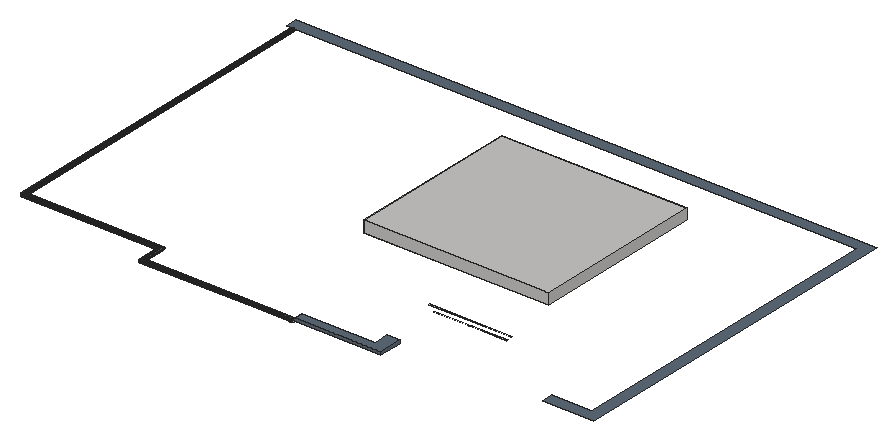
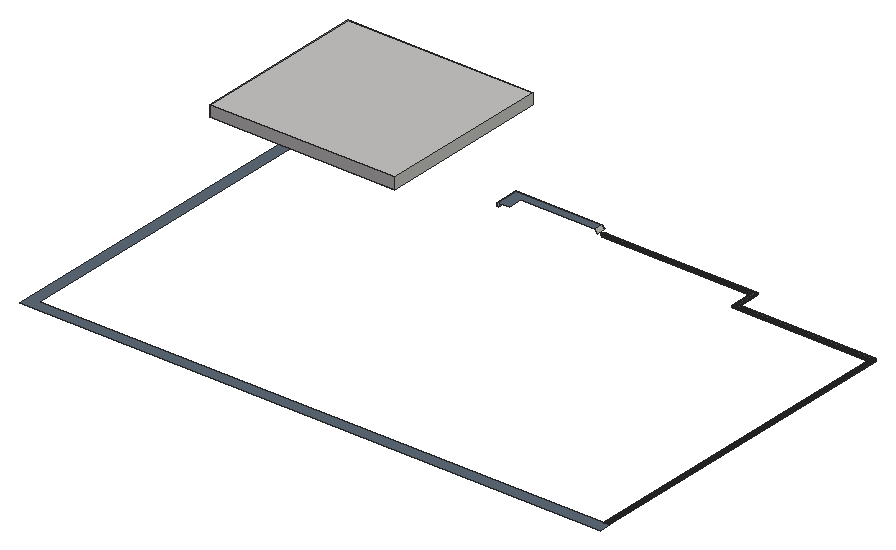
# SketchUp Ruby script. Lengths in inches.
U = 1.inch
M = Sketchup.active_model
def pt(a) = Geom::Point3d.new(a.map { |v| v * U })
def face(e, loops, mat)
  f = e.add_face(loops[0].map { |a| pt(a) })
  loops[1..].each { |l| e.add_face(l.map { |a| pt(a) }).erase! }
  f.material = f.back_material = mat if mat
  f
end
# faces: each face lists its corners as indices into pts; further lists are holes
def faces(e, pts, list, mat = nil) = list.each { |f| face(e, (f[0].is_a?(Array) ? f : [f]).map { |l| l.map { |i| pts[i] } }, mat) }
# xy, xz, yz: faces in a plane at the given z, y or x. An outline is a flat list of corners, or four numbers for a rectangle; further outlines are holes
def ring(l) = l.size == 4 ? [[l[0], l[1]], [l[2], l[1]], [l[2], l[3]], [l[0], l[3]]] : l.each_slice(2).to_a
def flat(e, list, mat, &to3) = list.each { |f| face(e, (f[0].is_a?(Array) ? f : [f]).map { |l| ring(l).map { |u, v| to3.(u, v) } }, mat) }
def xy(e, z, list, mat = nil) = flat(e, list, mat) { |x, y| [x, y, z] }
def xz(e, y, list, mat = nil) = flat(e, list, mat) { |x, z| [x, y, z] }
def yz(e, x, list, mat = nil) = flat(e, list, mat) { |y, z| [x, y, z] }
def lines(e, pts, list) = list.each { |a, b| e.add_line(pt(pts[a]), pt(pts[b])) }
# prism: a flat outline (further loops are holes) pulled along v
def prism(e, loops, v, mat = nil)
  f = face(e, loops, mat); d = Geom::Vector3d.new(v.map { |x| x * U })
  f.pushpull(f.normal.samedirection?(d) ? d.length : -d.length)
end
def box(e, o, s, mat = nil) = prism(e, [[o, [o[0] + s[0], o[1], o[2]], [o[0] + s[0], o[1] + s[1], o[2]], [o[0], o[1] + s[1], o[2]]]], [0, 0, s[2]], mat)
def at(x, y, z, deg = 0) = Geom::Transformation.translation(pt([x, y, z])) * Geom::Transformation.rotation(ORIGIN, Z_AXIS, deg.degrees)
def axes(o, x, y, z) = Geom::Transformation.new([*x, 0, *y, 0, *z, 0, *pt(o).to_a, 1])
def part(name) = M.definitions.add(name)
# library, detail: a bought-in or finely detailed component or shape, given as its bounding box
def library(name, o, s) = part(name).tap { |d| box(d.entities, o, s) }
def detail(e, o, s) = box(e.add_group.entities, o, s)
def put(e, d, t, mat = nil) = e.add_instance(d, t).tap { |i| i.material = mat if mat }
def group(e, t, mat = nil) = e.add_group.tap { |g| g.transformation = t; g.material = mat if mat }.entities
root = M.entities
M.materials.add("[0010_Snow]").color = [198, 195, 195]
M.materials.add("[0040_Peru]").color = [191, 124, 58]
M.materials.add("[0111_SlateGray]").color = [93, 106, 119]
xy(root,726,[[864,63,948,63,948,639,0,639,0,621,930,621,930,81,864,81]],"[0111_SlateGray]")
xy(root,726.875,[[485.39,25,485.39,27,627.8125,27,627.8125,63,629.8125,63,629.8125,25]],"[0111_SlateGray]")
xy(root,732,[[489.79,25,629.8125,25,629.8125,63,609.8125,63,609.8125,39,489.79,39]],"[0111_SlateGray]")
xy(root,793.97,[[687,62,746.59,63],[746.59,62,806.18,63]])
xy(root,801.97,[[679,62,814.18,63]])
xy(root,882,[[668.51,51.99,667.48,52.125,666.51,52.53,665.68,53.16,665.05,53.99,664.65,54.96,664.51,55.99,664.65,57.03,665.05,57.99,665.68,58.82,666.51,59.45,667.48,59.85,668.51,59.99,669.55,59.85,670.51,59.45,671.34,58.82,671.97,57.99,672.375,57.03,672.51,55.99,672.375,54.96,671.97,53.99,671.34,53.16,670.51,52.53,669.55,52.125],[728.51,51.99,727.48,52.125,726.51,52.53,725.68,53.16,725.05,53.99,724.65,54.96,724.51,55.99,724.65,57.03,725.05,57.99,725.68,58.82,726.51,59.45,727.48,59.85,728.51,59.99,729.55,59.85,730.51,59.45,731.34,58.82,731.97,57.99,732.375,57.03,732.51,55.99,732.375,54.96,731.97,53.99,731.34,53.16,730.51,52.53,729.55,52.125],[788.51,51.99,787.48,52.125,786.51,52.53,785.68,53.16,785.05,53.99,784.65,54.96,784.51,55.99,784.65,57.03,785.05,57.99,785.68,58.82,786.51,59.45,787.48,59.85,788.51,59.99,789.55,59.85,790.51,59.45,791.34,58.82,791.97,57.99,792.375,57.03,792.51,55.99,792.375,54.96,791.97,53.99,791.34,53.16,790.51,52.53,789.55,52.125],[609.8125,63,609.8125,303,621.8125,303,621.8125,81,852,81,852,303,864,303,864,63],[874.9375,71.95,873.375,72.05,871.89,72.55,870.59,73.42,869.55,74.59,868.86,76,868.55,77.53,868.65,79.09,869.15,80.58,870.01,81.88,871.1875,82.92,872.59,83.61,874.13,83.92,875.69,83.82,877.18,83.32,878.48,82.46,879.51,81.28,880.21,79.875,880.52,78.34,880.42,76.78,879.92,75.29,879.05,73.99,877.875,72.95,876.47,72.26],
  [597.26,71.99,595.71,72.19,594.26,72.79,593.02,73.74,592.07,74.99,591.47,76.43,591.26,77.99,591.47,79.54,592.07,80.99,593.02,82.23,594.26,83.18,595.71,83.78,597.26,83.99,598.82,83.78,600.26,83.18,601.51,82.23,602.46,80.99,603.06,79.54,603.26,77.99,603.06,76.43,602.46,74.99,601.51,73.74,600.26,72.79,598.82,72.19],[874.9375,107.95,873.375,108.05,871.89,108.55,870.59,109.42,869.55,110.59,868.86,112,868.55,113.53,868.65,115.09,869.15,116.58,870.01,117.88,871.1875,118.92,872.59,119.61,874.13,119.92,875.69,119.82,877.18,119.32,878.48,118.46,879.51,117.28,880.21,115.875,880.52,114.34,880.42,112.78,879.92,111.29,879.05,109.99,877.875,108.95,876.47,108.26],[597.26,107.99,595.71,108.19,594.26,108.79,593.02,109.74,592.07,110.99,591.47,112.43,591.26,113.99,591.47,115.54,592.07,116.99,593.02,118.23,594.26,119.18,595.71,119.78,597.26,119.99,598.82,119.78,600.26,119.18,601.51,118.23,602.46,116.99,603.06,115.54,603.26,113.99,603.06,112.43,602.46,110.99,601.51,109.74,600.26,108.79,598.82,108.19],[874.9375,143.95,873.375,144.05,871.89,144.55,870.59,145.42,869.55,146.59,868.86,148,868.55,149.53,868.65,151.09,869.15,152.58,870.01,153.88,871.1875,154.92,872.59,155.61,874.13,155.92,875.69,155.82,877.18,155.32,878.48,154.46,879.51,153.28,880.21,151.875,880.52,150.34,880.42,148.78,879.92,147.29,879.05,145.99,877.875,144.95,876.47,144.26],[597.26,143.99,595.71,144.19,594.26,144.79,593.02,145.74,592.07,146.99,591.47,148.43,591.26,149.99,591.47,151.54,592.07,152.99,593.02,154.23,594.26,155.18,595.71,155.78,597.26,155.99,598.82,155.78,600.26,155.18,601.51,154.23,602.46,152.99,603.06,151.54,603.26,149.99,603.06,148.43,602.46,146.99,601.51,145.74,600.26,144.79,598.82,144.19],
  [874.9375,179.95,873.375,180.05,871.89,180.55,870.59,181.42,869.55,182.59,868.86,184,868.55,185.53,868.65,187.09,869.15,188.58,870.01,189.88,871.1875,190.92,872.59,191.61,874.13,191.92,875.69,191.82,877.18,191.32,878.48,190.46,879.51,189.28,880.21,187.875,880.52,186.34,880.42,184.78,879.92,183.29,879.05,181.99,877.875,180.95,876.47,180.26],[597.26,179.99,595.71,180.19,594.26,180.79,593.02,181.74,592.07,182.99,591.47,184.43,591.26,185.99,591.47,187.54,592.07,188.99,593.02,190.23,594.26,191.18,595.71,191.78,597.26,191.99,598.82,191.78,600.26,191.18,601.51,190.23,602.46,188.99,603.06,187.54,603.26,185.99,603.06,184.43,602.46,182.99,601.51,181.74,600.26,180.79,598.82,180.19],[874.9375,215.95,873.375,216.05,871.89,216.55,870.59,217.42,869.55,218.59,868.86,220,868.55,221.53,868.65,223.09,869.15,224.58,870.01,225.88,871.1875,226.92,872.59,227.61,874.13,227.92,875.69,227.82,877.18,227.32,878.48,226.46,879.51,225.28,880.21,223.875,880.52,222.34,880.42,220.78,879.92,219.29,879.05,217.99,877.875,216.95,876.47,216.26],[597.26,215.99,595.71,216.19,594.26,216.79,593.02,217.74,592.07,218.99,591.47,220.43,591.26,221.99,591.47,223.54,592.07,224.99,593.02,226.23,594.26,227.18,595.71,227.78,597.26,227.99,598.82,227.78,600.26,227.18,601.51,226.23,602.46,224.99,603.06,223.54,603.26,221.99,603.06,220.43,602.46,218.99,601.51,217.74,600.26,216.79,598.82,216.19],[874.9375,251.95,873.375,252.05,871.89,252.55,870.59,253.42,869.55,254.59,868.86,256,868.55,257.53,868.65,259.09,869.15,260.58,870.01,261.88,871.1875,262.92,872.59,263.61,874.13,263.92,875.69,263.82,877.18,263.32,878.48,262.46,879.51,261.28,880.21,259.875,880.52,258.34,880.42,256.78,879.92,255.29,879.05,253.99,877.875,252.95,876.47,252.26],
  [597.26,251.99,595.71,252.19,594.26,252.79,593.02,253.74,592.07,254.99,591.47,256.43,591.26,257.99,591.47,259.54,592.07,260.99,593.02,262.23,594.26,263.18,595.71,263.78,597.26,263.99,598.82,263.78,600.26,263.18,601.51,262.23,602.46,260.99,603.06,259.54,603.26,257.99,603.06,256.43,602.46,254.99,601.51,253.74,600.26,252.79,598.82,252.19]])
xy(root,882,[[[585.8125,45,888,327],[609.8125,63,864,63,864,303,852,303,852,81,621.8125,81,621.8125,303,609.8125,303],[874.9375,71.95,876.47,72.26,877.875,72.95,879.05,73.99,879.92,75.29,880.42,76.78,880.52,78.34,880.21,79.875,879.51,81.28,878.48,82.46,877.18,83.32,875.69,83.82,874.13,83.92,872.59,83.61,871.1875,82.92,870.01,81.88,869.15,80.58,868.65,79.09,868.55,77.53,868.86,76,869.55,74.59,870.59,73.42,871.89,72.55,873.375,72.05],[874.9375,107.95,876.47,108.26,877.875,108.95,879.05,109.99,879.92,111.29,880.42,112.78,880.52,114.34,880.21,115.875,879.51,117.28,878.48,118.46,877.18,119.32,875.69,119.82,874.13,119.92,872.59,119.61,871.1875,118.92,870.01,117.88,869.15,116.58,868.65,115.09,868.55,113.53,868.86,112,869.55,110.59,870.59,109.42,871.89,108.55,873.375,108.05],[874.9375,179.95,876.47,180.26,877.875,180.95,879.05,181.99,879.92,183.29,880.42,184.78,880.52,186.34,880.21,187.875,879.51,189.28,878.48,190.46,877.18,191.32,875.69,191.82,874.13,191.92,872.59,191.61,871.1875,190.92,870.01,189.88,869.15,188.58,868.65,187.09,868.55,185.53,868.86,184,869.55,182.59,870.59,181.42,871.89,180.55,873.375,180.05],[874.9375,143.95,876.47,144.26,877.875,144.95,879.05,145.99,879.92,147.29,880.42,148.78,880.52,150.34,880.21,151.875,879.51,153.28,878.48,154.46,877.18,155.32,875.69,155.82,874.13,155.92,872.59,155.61,871.1875,154.92,870.01,153.88,869.15,152.58,868.65,151.09,868.55,149.53,868.86,148,869.55,146.59,870.59,145.42,871.89,144.55,873.375,144.05],[874.9375,215.95,876.47,216.26,877.875,216.95,879.05,217.99,879.92,219.29,880.42,220.78,880.52,222.34,880.21,223.875,879.51,225.28,878.48,226.46,877.18,227.32,875.69,227.82,874.13,227.92,872.59,227.61,871.1875,226.92,870.01,225.88,869.15,224.58,868.65,223.09,868.55,221.53,868.86,220,869.55,218.59,870.59,217.42,871.89,216.55,873.375,216.05],[874.9375,251.95,876.47,252.26,877.875,252.95,879.05,253.99,879.92,255.29,880.42,256.78,880.52,258.34,880.21,259.875,879.51,261.28,878.48,262.46,877.18,263.32,875.69,263.82,874.13,263.92,872.59,263.61,871.1875,262.92,870.01,261.88,869.15,260.58,868.65,259.09,868.55,257.53,868.86,256,869.55,254.59,870.59,253.42,871.89,252.55,873.375,252.05],[597.26,143.99,598.82,144.19,600.26,144.79,601.51,145.74,602.46,146.99,603.06,148.43,603.26,149.99,603.06,151.54,602.46,152.99,601.51,154.23,600.26,155.18,598.82,155.78,597.26,155.99,595.71,155.78,594.26,155.18,593.02,154.23,592.07,152.99,591.47,151.54,591.26,149.99,591.47,148.43,592.07,146.99,593.02,145.74,594.26,144.79,595.71,144.19],[597.26,71.99,598.82,72.19,600.26,72.79,601.51,73.74,602.46,74.99,603.06,76.43,603.26,77.99,603.06,79.54,602.46,80.99,601.51,82.23,600.26,83.18,598.82,83.78,597.26,83.99,595.71,83.78,594.26,83.18,593.02,82.23,592.07,80.99,591.47,79.54,591.26,77.99,591.47,76.43,592.07,74.99,593.02,73.74,594.26,72.79,595.71,72.19],[597.26,107.99,598.82,108.19,600.26,108.79,601.51,109.74,602.46,110.99,603.06,112.43,603.26,113.99,603.06,115.54,602.46,116.99,601.51,118.23,600.26,119.18,598.82,119.78,597.26,119.99,595.71,119.78,594.26,119.18,593.02,118.23,592.07,116.99,591.47,115.54,591.26,113.99,591.47,112.43,592.07,110.99,593.02,109.74,594.26,108.79,595.71,108.19],[597.26,179.99,598.82,180.19,600.26,180.79,601.51,181.74,602.46,182.99,603.06,184.43,603.26,185.99,603.06,187.54,602.46,188.99,601.51,190.23,600.26,191.18,598.82,191.78,597.26,191.99,595.71,191.78,594.26,191.18,593.02,190.23,592.07,188.99,591.47,187.54,591.26,185.99,591.47,184.43,592.07,182.99,593.02,181.74,594.26,180.79,595.71,180.19],[597.26,215.99,598.82,216.19,600.26,216.79,601.51,217.74,602.46,218.99,603.06,220.43,603.26,221.99,603.06,223.54,602.46,224.99,601.51,226.23,600.26,227.18,598.82,227.78,597.26,227.99,595.71,227.78,594.26,227.18,593.02,226.23,592.07,224.99,591.47,223.54,591.26,221.99,591.47,220.43,592.07,218.99,593.02,217.74,594.26,216.79,595.71,216.19],[597.26,251.99,598.82,252.19,600.26,252.79,601.51,253.74,602.46,254.99,603.06,256.43,603.26,257.99,603.06,259.54,602.46,260.99,601.51,262.23,600.26,263.18,598.82,263.78,597.26,263.99,595.71,263.78,594.26,263.18,593.02,262.23,592.07,260.99,591.47,259.54,591.26,257.99,591.47,256.43,592.07,254.99,593.02,253.74,594.26,252.79,595.71,252.19],[728.51,51.99,729.55,52.125,730.51,52.53,731.34,53.16,731.97,53.99,732.375,54.96,732.51,55.99,732.375,57.03,731.97,57.99,731.34,58.82,730.51,59.45,729.55,59.85,728.51,59.99,727.48,59.85,726.51,59.45,725.68,58.82,725.05,57.99,724.65,57.03,724.51,55.99,724.65,54.96,725.05,53.99,725.68,53.16,726.51,52.53,727.48,52.125],[788.51,51.99,789.55,52.125,790.51,52.53,791.34,53.16,791.97,53.99,792.375,54.96,792.51,55.99,792.375,57.03,791.97,57.99,791.34,58.82,790.51,59.45,789.55,59.85,788.51,59.99,787.48,59.85,786.51,59.45,785.68,58.82,785.05,57.99,784.65,57.03,784.51,55.99,784.65,54.96,785.05,53.99,785.68,53.16,786.51,52.53,787.48,52.125],[668.51,51.99,669.55,52.125,670.51,52.53,671.34,53.16,671.97,53.99,672.375,54.96,672.51,55.99,672.375,57.03,671.97,57.99,671.34,58.82,670.51,59.45,669.55,59.85,668.51,59.99,667.48,59.85,666.51,59.45,665.68,58.82,665.05,57.99,664.65,57.03,664.51,55.99,664.65,54.96,665.05,53.99,665.68,53.16,666.51,52.53,667.48,52.125]]],"[0040_Peru]")
xy(root,900,[[585.8125,45,888,327]],"[0010_Snow]")
xz(root,25,[[485.39,726.875,629.8125,726.875,629.8125,732,489.79,732]],"[0111_SlateGray]")
xz(root,45,[[585.8125,882,888,900]],"[0010_Snow]")
xz(root,63,[[627.8125,726.875,629.8125,732]])
xz(root,327,[[585.8125,882,888,900]],"[0010_Snow]")
xz(root,621,[[9,720,8.6875,720.02,8.375,720.07,8.07,720.15,7.78,720.26,7.5,720.4,7.24,720.57,6.99,720.77,6.77,720.99,6.57,721.24,6.4,721.5,6.26,721.78,6.15,722.07,6.07,722.375,6.02,722.6875,6,723,6.02,723.3125,6.07,723.625,6.15,723.93,6.26,724.22,6.4,724.5,6.57,724.76,6.77,725.01,6.99,725.23,7.24,725.43,7.5,725.6,7.78,725.74,8.07,725.85,8.375,725.93,8.6875,725.98,9,726,9.3125,725.98,9.625,725.93,9.93,725.85,10.22,725.74,10.5,725.6,10.76,725.43,11.01,725.23,11.23,725.01,11.43,724.76,11.6,724.5,11.74,724.22,11.85,723.93,11.93,723.625,11.98,723.3125,12,723,11.98,722.6875,11.93,722.375,11.85,722.07,11.74,721.78,11.6,721.5,11.43,721.24,11.23,720.99,11.01,720.77,10.76,720.57,10.5,720.4,10.22,720.26,9.93,720.15,9.625,720.07,9.3125,720.02]])
yz(root,482.06,[[32,720,32.3125,720.02,32.625,720.07,32.93,720.15,33.22,720.26,33.5,720.4,33.76,720.57,34.01,720.77,34.23,720.99,34.43,721.24,34.6,721.5,34.74,721.78,34.85,722.07,34.93,722.375,34.98,722.6875,35,723,34.98,723.3125,34.93,723.625,34.85,723.93,34.74,724.22,34.6,724.5,34.43,724.76,34.23,725.01,34.01,725.23,33.76,725.43,33.5,725.6,33.22,725.74,32.93,725.85,32.625,725.93,32.3125,725.98,32,726,31.6875,725.98,31.375,725.93,31.07,725.85,30.78,725.74,30.5,725.6,30.24,725.43,29.99,725.23,29.77,725.01,29.57,724.76,29.4,724.5,29.26,724.22,29.15,723.93,29.07,723.625,29.02,723.3125,29,723,29.02,722.6875,29.07,722.375,29.15,722.07,29.26,721.78,29.4,721.5,29.57,721.24,29.77,720.99,29.99,720.77,30.24,720.57,30.5,720.4,30.78,720.26,31.07,720.15,31.375,720.07,31.6875,720.02]])
yz(root,585.8125,[[45,882,327,900]])
yz(root,629.8125,[[25,726.875,63,732]],"[0111_SlateGray]")
yz(root,888,[[45,882,327,900]],"[0010_Snow]")
p = [[233.375,71.375,720.07],[233.6875,71.6875,720.02],[233.6875,31.6875,720.02],[233.375,31.375,720.07],[482.06,31.6875,720.02],[482.06,31.375,720.07],
  [234,72,720],[234,32,720],[482.06,32,720],[234.3125,72.3125,720.02],[234.3125,32.3125,720.02],[482.06,32.3125,720.02],
  [234.625,72.625,720.07],[234.625,32.625,720.07],[482.06,32.625,720.07],[8.375,621,720.07],[8.6875,621,720.02],[8.6875,71.6875,720.02],
  [8.375,71.375,720.07],[9,621,720],[9,72,720],[9.3125,621,720.02],[9.3125,72.3125,720.02],[9.625,621,720.07],
  [9.625,72.625,720.07],[232.78,70.78,720.26],[233.07,71.07,720.15],[233.07,31.07,720.15],[232.78,30.78,720.26],[482.06,31.07,720.15],
  [482.06,30.78,720.26],[234.93,72.93,720.15],[234.93,32.93,720.15],[482.06,32.93,720.15],[235.22,73.22,720.26],[235.22,33.22,720.26],
  [482.06,33.22,720.26],[7.78,621,720.26],[8.07,621,720.15],[8.07,71.07,720.15],[7.78,70.78,720.26],[9.93,621,720.15],
  [9.93,72.93,720.15],[10.22,621,720.26],[10.22,73.22,720.26],[232.5,70.5,720.4],[232.5,30.5,720.4],[482.06,30.5,720.4],
  [235.5,73.5,720.4],[235.5,33.5,720.4],[482.06,33.5,720.4],[7.5,621,720.4],[7.5,70.5,720.4],[10.5,621,720.4],
  [10.5,73.5,720.4],[232.24,70.24,720.57],[232.24,30.24,720.57],[482.06,30.24,720.57],[235.76,73.76,720.57],[235.76,33.76,720.57],
  [482.06,33.76,720.57],[7.24,621,720.57],[7.24,70.24,720.57],[10.76,621,720.57],[10.76,73.76,720.57],[231.99,69.99,720.77],
  [231.99,29.99,720.77],[482.06,29.99,720.77],[236.01,74.01,720.77],[236.01,34.01,720.77],[482.06,34.01,720.77],[6.99,621,720.77],
  [6.99,69.99,720.77],[11.01,621,720.77],[11.01,74.01,720.77],[483.86,33.16,725.1],[483.77,33.45,724.99],[483.66,33.71,724.87],
  [483.53,33.96,724.72],[483.39,34.1875,724.56],[483.24,34.39,724.375],[483.07,34.57,724.18],[482.89,34.72,723.97],[482.7,34.83,723.75],
  [482.5,34.92,723.52],[482.3,34.98,723.28],[482.09,35,723.05],[481.89,34.99,722.81],[481.6875,34.95,722.57],[481.49,34.87,722.34],
  [481.3,34.76,722.12],[481.11,34.63,721.9],[480.9375,34.46,721.7],[480.78,34.27,721.51],[480.63,34.05,721.34],[480.5,33.8125,721.1875],
  [480.38,33.55,721.05],[480.29,33.28,720.94],[480.21,32.98,720.85],[480.15,32.68,720.78],[480.11,32.375,720.74],[480.1,32.06,720.73],
  [480.11,31.75,720.73],[480.13,31.4375,720.77],[480.18,31.13,720.82],[480.25,30.84,720.9],[480.34,30.55,721.01],[480.45,30.29,721.13],
  [480.58,30.04,721.28],[480.72,29.8125,721.44],[480.875,29.61,721.625],[481.04,29.43,721.82],[481.22,29.28,722.03],[481.41,29.17,722.25],
  [481.61,29.08,722.48],[481.8125,29.02,722.72],[482.02,29,722.95],[482.22,29.01,723.19],[482.42,29.05,723.43],[482.62,29.13,723.66],
  [482.8125,29.24,723.88],[483,29.37,724.1],[483.17,29.54,724.3],[483.33,29.73,724.49],[483.48,29.95,724.66],[483.61,30.1875,724.8125],
  [483.73,30.45,724.95],[483.83,30.72,725.06],[483.9,31.02,725.15],[483.96,31.32,725.22],[484,31.625,725.26],[484.01,31.94,725.27],
  [484,32.25,725.27],[483.98,32.5625,725.23],[483.93,32.87,725.18],[231.77,69.77,720.99],[231.77,29.77,720.99],[482.06,29.77,720.99],
  [236.23,74.23,720.99],[236.23,34.23,720.99],[482.06,34.23,720.99],[6.77,621,720.99],[6.77,69.77,720.99],[11.23,621,720.99],
  [11.23,74.23,720.99],[231.57,69.57,721.24],[231.57,29.57,721.24],[482.06,29.57,721.24],[236.43,74.43,721.24],[236.43,34.43,721.24],
  [482.06,34.43,721.24],[6.57,621,721.24],[6.57,69.57,721.24],[11.43,621,721.24],[11.43,74.43,721.24],[231.4,69.4,721.5],
  [231.4,29.4,721.5],[482.06,29.4,721.5],[236.6,74.6,721.5],[236.6,34.6,721.5],[482.06,34.6,721.5],[6.4,621,721.5],
  [6.4,69.4,721.5],[11.6,621,721.5],[11.6,74.6,721.5],[231.26,69.26,721.78],[231.26,29.26,721.78],[482.06,29.26,721.78],
  [236.74,74.74,721.78],[236.74,34.74,721.78],[482.06,34.74,721.78],[6.26,621,721.78],[6.26,69.26,721.78],[11.74,621,721.78],
  [11.74,74.74,721.78],[231.15,69.15,722.07],[231.15,29.15,722.07],[482.06,29.15,722.07],[236.85,74.85,722.07],[236.85,34.85,722.07],
  [482.06,34.85,722.07],[6.15,621,722.07],[6.15,69.15,722.07],[11.85,621,722.07],[11.85,74.85,722.07],[231.07,69.07,722.375],
  [231.07,29.07,722.375],[482.06,29.07,722.375],[236.93,74.93,722.375],[236.93,34.93,722.375],[482.06,34.93,722.375],[6.07,621,722.375],
  [6.07,69.07,722.375],[11.93,621,722.375],[11.93,74.93,722.375],[231.02,69.02,722.6875],[231.02,29.02,722.6875],[482.06,29.02,722.6875],
  [236.98,74.98,722.6875],[236.98,34.98,722.6875],[482.06,34.98,722.6875],[6.02,621,722.6875],[6.02,69.02,722.6875],[11.98,621,722.6875],
  [11.98,74.98,722.6875],[231,69,723],[231,29,723],[482.06,29,723],[237,75,723],[237,35,723],
  [482.06,35,723],[6,621,723],[6,69,723],[12,621,723],[12,75,723],[231.02,69.02,723.3125],
  [231.02,29.02,723.3125],[482.06,29.02,723.3125],[236.98,74.98,723.3125],[236.98,34.98,723.3125],[482.06,34.98,723.3125],[6.02,621,723.3125],
  [6.02,69.02,723.3125],[11.98,621,723.3125],[11.98,74.98,723.3125],[231.07,69.07,723.625],[231.07,29.07,723.625],[482.06,29.07,723.625],
  [236.93,74.93,723.625],[236.93,34.93,723.625],[482.06,34.93,723.625],[6.07,621,723.625],[6.07,69.07,723.625],[11.93,621,723.625],
  [11.93,74.93,723.625],[231.15,69.15,723.93],[231.15,29.15,723.93],[482.06,29.15,723.93],[236.85,74.85,723.93],[236.85,34.85,723.93],
  [482.06,34.85,723.93],[6.15,621,723.93],[6.15,69.15,723.93],[11.85,621,723.93],[11.85,74.85,723.93],[231.26,69.26,724.22],
  [231.26,29.26,724.22],[482.06,29.26,724.22],[236.74,74.74,724.22],[236.74,34.74,724.22],[482.06,34.74,724.22],[6.26,621,724.22],
  [6.26,69.26,724.22],[11.74,621,724.22],[11.74,74.74,724.22],[231.4,69.4,724.5],[231.4,29.4,724.5],[482.06,29.4,724.5],
  [236.6,74.6,724.5],[236.6,34.6,724.5],[482.06,34.6,724.5],[6.4,621,724.5],[6.4,69.4,724.5],[11.6,621,724.5],
  [11.6,74.6,724.5],[231.57,69.57,724.76],[231.57,29.57,724.76],[482.06,29.57,724.76],[236.43,74.43,724.76],[236.43,34.43,724.76],
  [482.06,34.43,724.76],[6.57,621,724.76],[6.57,69.57,724.76],[11.43,621,724.76],[11.43,74.43,724.76],[231.77,69.77,725.01],
  [231.77,29.77,725.01],[482.06,29.77,725.01],[236.23,74.23,725.01],[236.23,34.23,725.01],[482.06,34.23,725.01],[6.77,621,725.01],
  [6.77,69.77,725.01],[11.23,621,725.01],[11.23,74.23,725.01],[231.99,69.99,725.23],[231.99,29.99,725.23],[482.06,29.99,725.23],
  [236.01,74.01,725.23],[236.01,34.01,725.23],[482.06,34.01,725.23],[6.99,621,725.23],[6.99,69.99,725.23],[11.01,621,725.23],
  [11.01,74.01,725.23],[232.24,70.24,725.43],[232.24,30.24,725.43],[482.06,30.24,725.43],[235.76,73.76,725.43],[235.76,33.76,725.43],
  [482.06,33.76,725.43],[7.24,621,725.43],[7.24,70.24,725.43],[10.76,621,725.43],[10.76,73.76,725.43],[232.5,70.5,725.6],
  [232.5,30.5,725.6],[482.06,30.5,725.6],[235.5,73.5,725.6],[235.5,33.5,725.6],[482.06,33.5,725.6],[7.5,621,725.6],
  [7.5,70.5,725.6],[10.5,621,725.6],[10.5,73.5,725.6],[232.78,70.78,725.74],[232.78,30.78,725.74],[482.06,30.78,725.74],
  [235.22,73.22,725.74],[235.22,33.22,725.74],[482.06,33.22,725.74],[7.78,621,725.74],[7.78,70.78,725.74],[10.22,621,725.74],
  [10.22,73.22,725.74],[233.07,71.07,725.85],[233.07,31.07,725.85],[482.06,31.07,725.85],[234.93,72.93,725.85],[234.93,32.93,725.85],
  [482.06,32.93,725.85],[8.07,621,725.85],[8.07,71.07,725.85],[9.93,621,725.85],[9.93,72.93,725.85],[233.375,71.375,725.93],
  [233.375,31.375,725.93],[482.06,31.375,725.93],[233.6875,71.6875,725.98],[233.6875,31.6875,725.98],[482.06,31.6875,725.98],[234.625,72.625,725.93],
  [234.3125,72.3125,725.98],[234.3125,32.3125,725.98],[234.625,32.625,725.93],[482.06,32.3125,725.98],[482.06,32.625,725.93],[8.375,621,725.93],
  [8.375,71.375,725.93],[8.6875,621,725.98],[8.6875,71.6875,725.98],[9.625,621,725.93],[9.3125,621,725.98],[9.3125,72.3125,725.98],
  [9.625,72.625,725.93],[234,72,726],[234,32,726],[482.06,32,726],[9,621,726],[9,72,726],
  [489.79,25,732],[489.79,39,732],[485.39,39,726.875],[485.39,27,726.875],[485.39,25,726.875],[621.8125,81,882],
  [621.8125,81,900],[234,32,723],[482.06,32,723],[234,72,723],[9,72,723],[9,621,723]]
faces(root,p,[[0,1,2,3],[3,2,4,5],[1,6,7,2],[2,7,8,4],[6,9,10,7],[7,10,11,8],[9,12,13,10],[10,13,14,11],
  [15,16,17,18],[18,17,1,0],[16,19,20,17],[17,20,6,1],[19,21,22,20],[20,22,9,6],[21,23,24,22],[22,24,12,9],
  [25,26,27,28],[28,27,29,30],[26,0,3,27],[27,3,5,29],[12,31,32,13],[13,32,33,14],[31,34,35,32],[32,35,36,33],
  [37,38,39,40],[40,39,26,25],[38,15,18,39],[39,18,0,26],[23,41,42,24],[24,42,31,12],[41,43,44,42],[42,44,34,31],
  [45,25,28,46],[46,28,30,47],[34,48,49,35],[35,49,50,36],[51,37,40,52],[52,40,25,45],[43,53,54,44],[44,54,48,34],
  [55,45,46,56],[56,46,47,57],[48,58,59,49],[49,59,60,50],[61,51,52,62],[62,52,45,55],[53,63,64,54],[54,64,58,48],
  [65,55,56,66],[66,56,57,67],[58,68,69,59],[59,69,70,60],[71,61,62,72],[72,62,55,65],[63,73,74,64],[64,74,68,58],
  [135,65,66,136],[136,66,67,137],[68,138,139,69],[69,139,140,70],[141,71,72,142],[142,72,65,135],[73,143,144,74],[74,144,138,68],
  [145,135,136,146],[146,136,137,147],[138,148,149,139],[139,149,150,140],[151,141,142,152],[152,142,135,145],[143,153,154,144],[144,154,148,138],
  [155,145,146,156],[156,146,147,157],[148,158,159,149],[149,159,160,150],[161,151,152,162],[162,152,145,155],[153,163,164,154],[154,164,158,148],
  [165,155,156,166],[166,156,157,167],[158,168,169,159],[159,169,170,160],[171,161,162,172],[172,162,155,165],[163,173,174,164],[164,174,168,158],
  [175,165,166,176],[176,166,167,177],[168,178,179,169],[169,179,180,170],[181,171,172,182],[182,172,165,175],[173,183,184,174],[174,184,178,168],
  [185,175,176,186],[186,176,177,187],[178,188,189,179],[179,189,190,180],[191,181,182,192],[192,182,175,185],[183,193,194,184],[184,194,188,178],
  [195,185,186,196],[196,186,187,197],[188,198,199,189],[189,199,200,190],[201,191,192,202],[202,192,185,195],[193,203,204,194],[194,204,198,188],
  [205,195,196,206],[206,196,197,207],[198,208,209,199],[199,209,210,200],[211,201,202,212],[212,202,195,205],[203,213,214,204],[204,214,208,198],
  [215,205,206,216],[216,206,207,217],[208,218,219,209],[209,219,220,210],[221,211,212,222],[222,212,205,215],[213,223,224,214],[214,224,218,208],
  [225,215,216,226],[226,216,217,227],[218,228,229,219],[219,229,230,220],[231,221,222,232],[232,222,215,225],[223,233,234,224],[224,234,228,218],
  [235,225,226,236],[236,226,227,237],[228,238,239,229],[229,239,240,230],[241,231,232,242],[242,232,225,235],[233,243,244,234],[234,244,238,228],
  [245,235,236,246],[246,236,237,247],[238,248,249,239],[239,249,250,240],[251,241,242,252],[252,242,235,245],[243,253,254,244],[244,254,248,238],
  [255,245,246,256],[256,246,247,257],[248,258,259,249],[249,259,260,250],[261,251,252,262],[262,252,245,255],[253,263,264,254],[254,264,258,248],
  [265,255,256,266],[266,256,257,267],[258,268,269,259],[259,269,270,260],[271,261,262,272],[272,262,255,265],[263,273,274,264],[264,274,268,258],
  [275,265,266,276],[276,266,267,277],[268,278,279,269],[269,279,280,270],[281,271,272,282],[282,272,265,275],[273,283,284,274],[274,284,278,268],
  [285,275,276,286],[286,276,277,287],[278,288,289,279],[279,289,290,280],[291,281,282,292],[292,282,275,285],[283,293,294,284],[284,294,288,278],
  [295,285,286,296],[296,286,287,297],[288,298,299,289],[289,299,300,290],[301,291,292,302],[302,292,285,295],[293,303,304,294],[294,304,298,288],
  [305,295,296,306],[306,296,297,307],[298,308,309,299],[299,309,310,300],[311,301,302,312],[312,302,295,305],[303,313,314,304],[304,314,308,298],
  [315,305,306,316],[316,306,307,317],[308,318,319,309],[309,319,320,310],[321,311,312,322],[322,312,305,315],[313,323,324,314],[314,324,318,308],
  [325,315,316,326],[326,316,317,327],[318,328,329,319],[319,329,330,320],[331,321,322,332],[332,322,315,325],[323,333,334,324],[324,334,328,318],
  [335,325,326,336],[336,326,327,337],[338,335,336,339],[339,336,337,340],[341,342,343,344],[344,343,345,346],[328,341,344,329],[329,344,346,330],
  [347,331,332,348],[348,332,325,335],[349,347,348,350],[350,348,335,338],[351,352,353,354],[354,353,342,341],[333,351,354,334],[334,354,341,328],
  [355,338,339,356],[356,339,340,357],[342,355,356,343],[343,356,357,345],[358,349,350,359],[359,350,338,355],[352,358,359,353],[353,359,355,342]],"[0111_SlateGray]")
faces(root,p,[[75,76,77,78,79,80,81,82,83,84,85,86,87,88,89,90,91,92,93,94,95,96,97,98,99,100,101,102,103,104,105,106,107,108,109,110,111,112,113,114,115,116,117,118,119,120,121,122,123,124,125,126,127,128,129,130,131,132,133,134],[360,361,362,363,364]])
lines(root,p,[[365,366],[367,368],[367,369],[369,370],[370,371],[7,367],[6,369],[20,370]])
